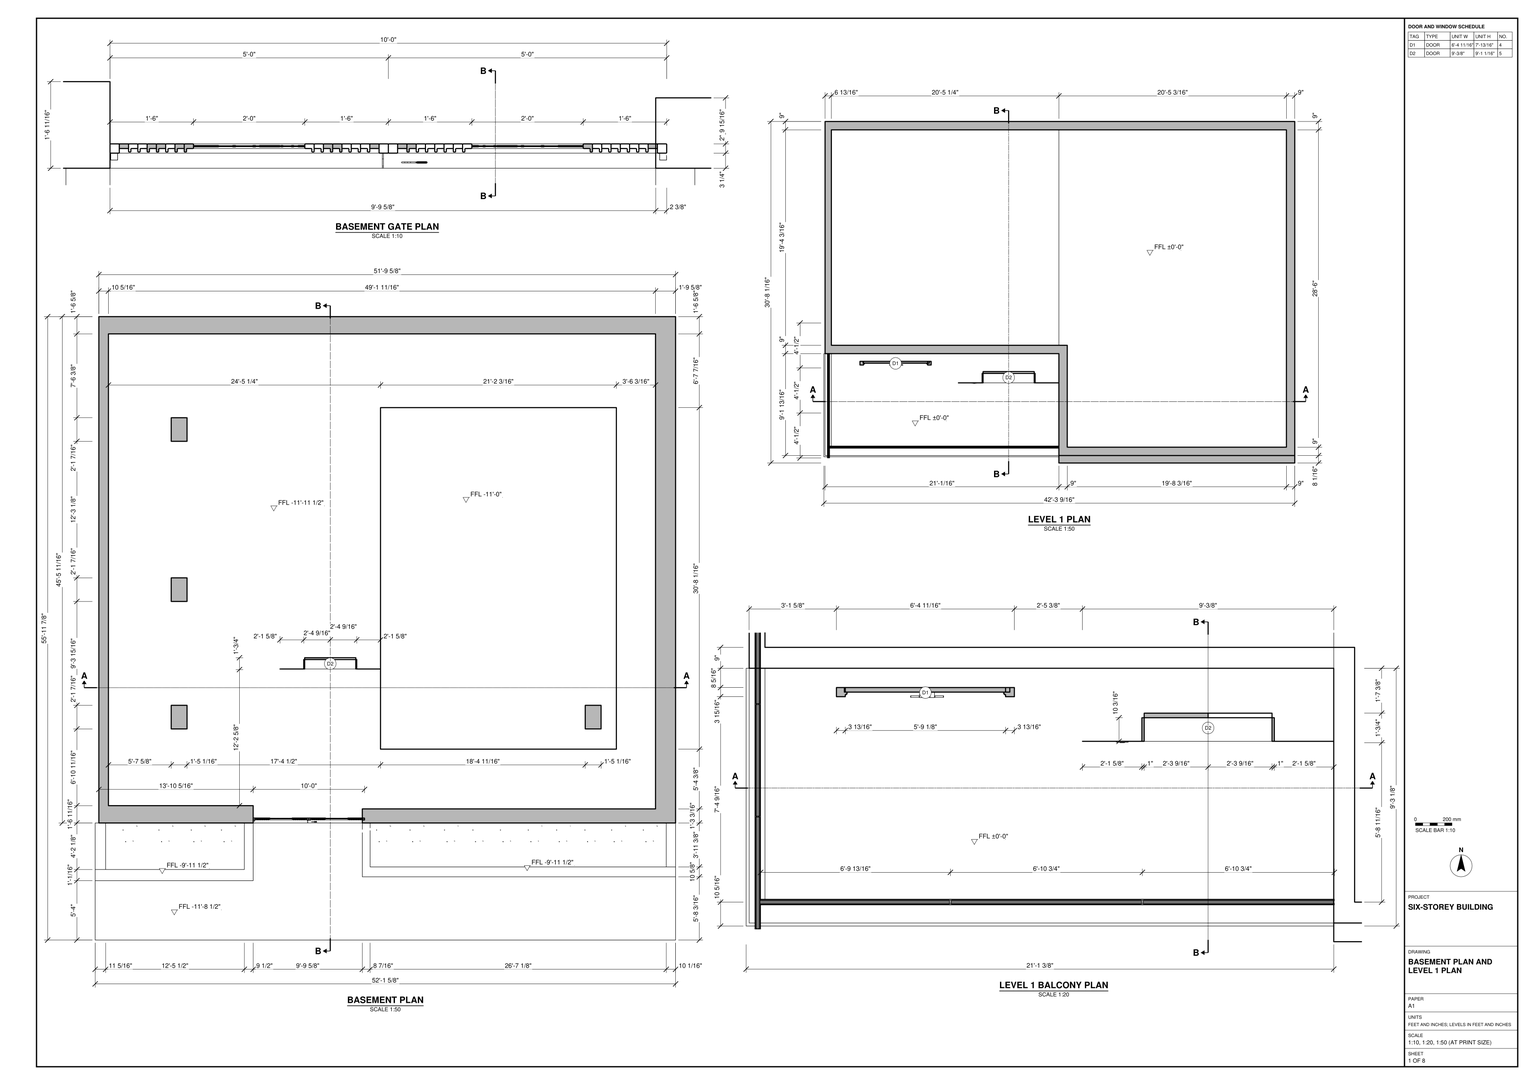
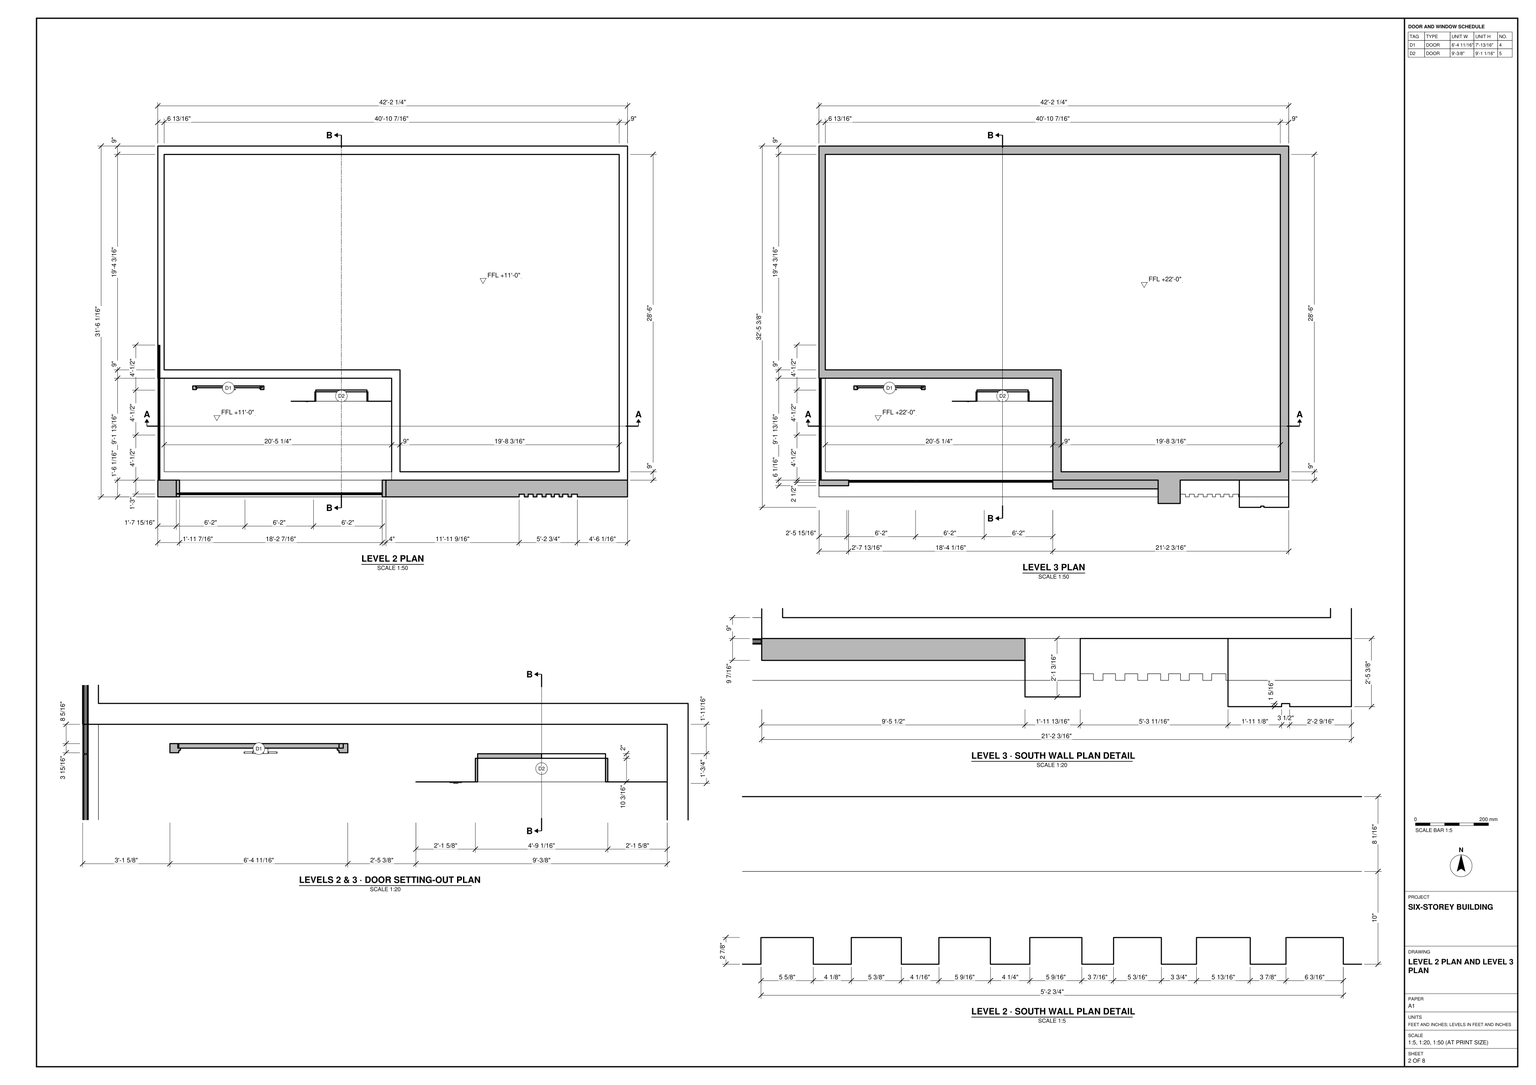
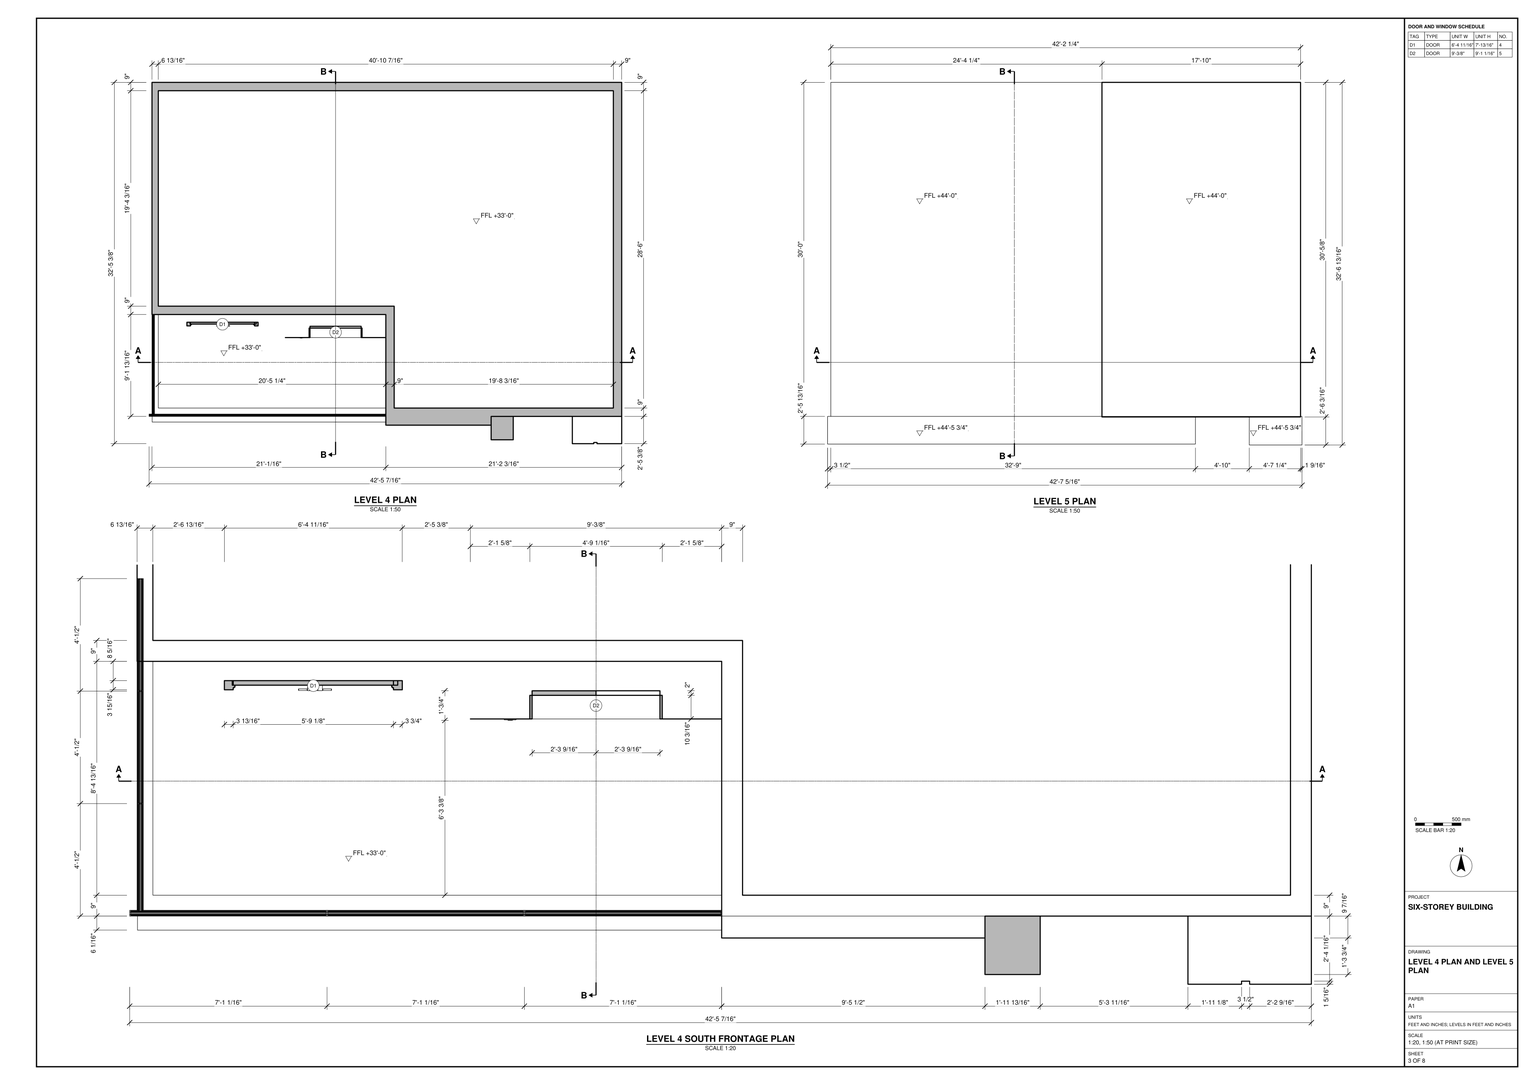
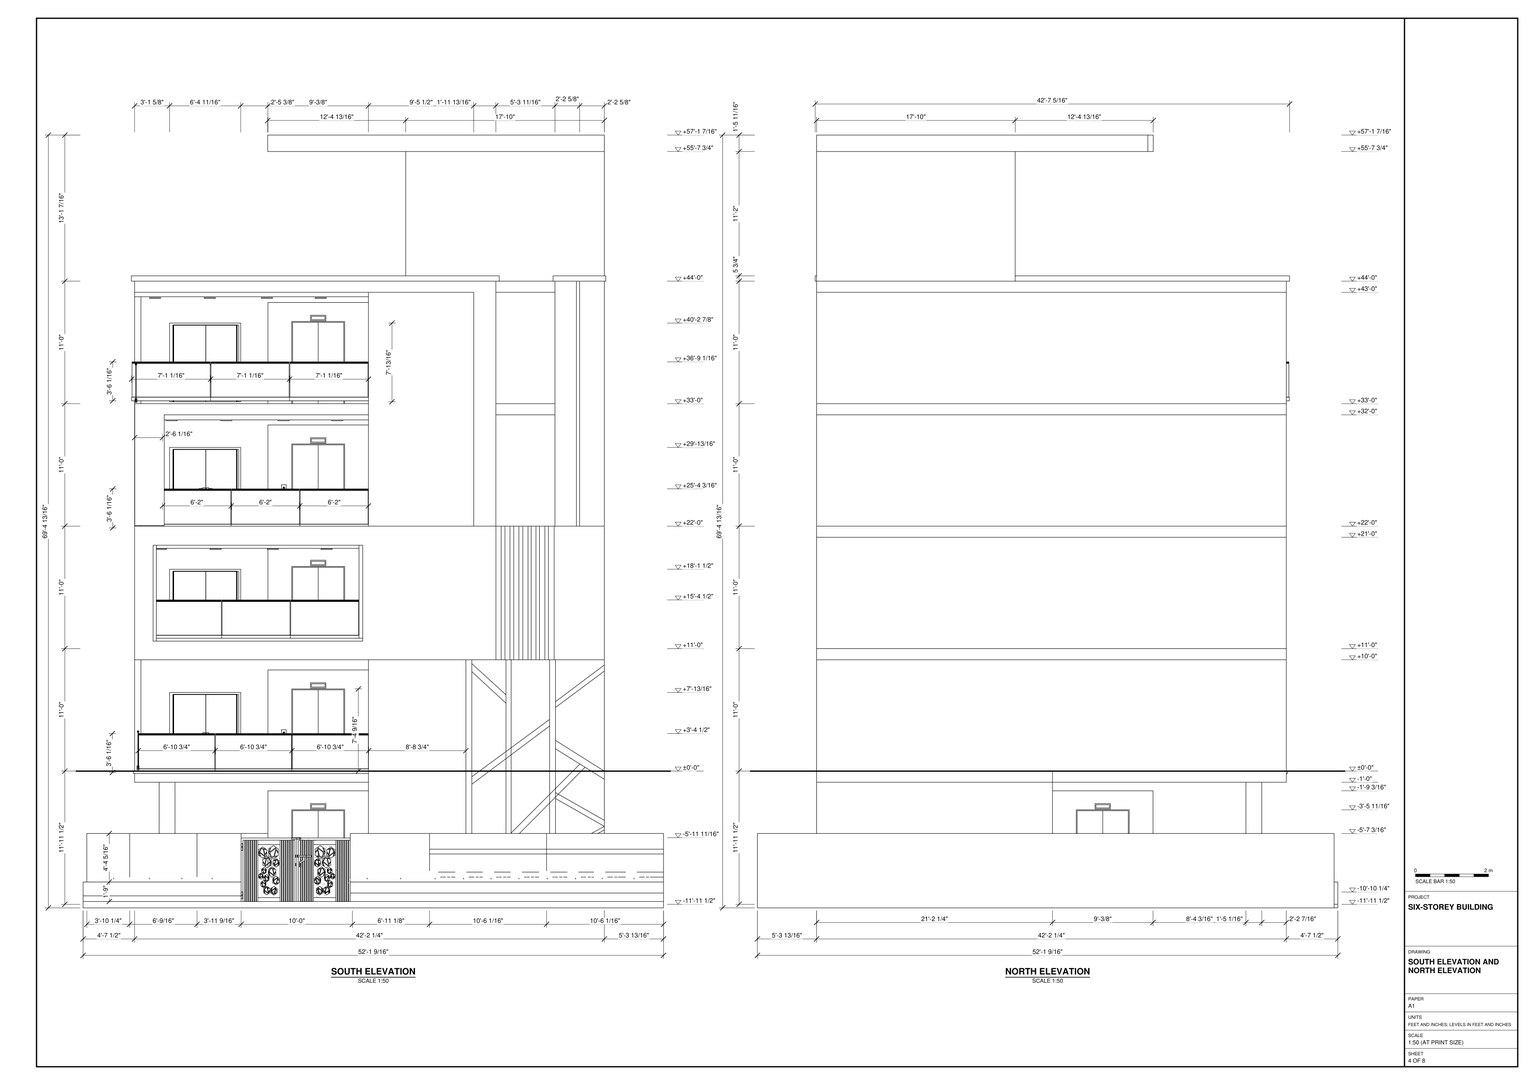
Work in feet and inches in SketchUp. Use the plans, sections, elevations and details in task_files/diagram_01.pdf. Set out the complete model at 52'-1 9/16" wide, 55'-11 7/8" deep and 69'-4 13/16" high, including the basement frontage. Use finished floor levels of -11'-11 1/2" for the basement, ±0'-0" for Level 1, +11'-0" for Level 2, +22'-0" for Level 3, +33'-0" for Level 4 and +44'-0" for Level 5.

Start with the basement perimeter, floor slabs, columns and gated opening in the south wall. Above the basement, follow the wall thicknesses and slab outlines on each plan. On Levels 1 through 4, set the balcony back into the west half of the south frontage. Place the paired entrance doors and lift doors according to the balcony details, and model the glazed balcony rails. Follow the changes in the projecting wall sections and ribbed detail on the east half of the frontage rather than copying one facade up the building. Finish the roof slabs to the outlines and heights on the Level 5 plan.

Keep shell elements such as walls, slabs and roof sections in separate groups or components, and do the same for each furniture or joinery piece shown. Use components for repeated parts. Decor and loose items may be any suitable library components. Save one SketchUp model as output_files/six_storey_building_with_recessed_balconies.skp.

# SketchUp Ruby script. Lengths in inches.
U = 1.inch
M = Sketchup.active_model
def pt(a) = Geom::Point3d.new(a.map { |v| v * U })
def face(e, loops, mat)
  f = e.add_face(loops[0].map { |a| pt(a) })
  loops[1..].each { |l| e.add_face(l.map { |a| pt(a) }).erase! }
  f.material = f.back_material = mat if mat
  f
end
# faces: each face lists its corners as indices into pts; further lists are holes
def faces(e, pts, list, mat = nil) = list.each { |f| face(e, (f[0].is_a?(Array) ? f : [f]).map { |l| l.map { |i| pts[i] } }, mat) }
# xy, xz, yz: faces in a plane at the given z, y or x. An outline is a flat list of corners, or four numbers for a rectangle; further outlines are holes
def ring(l) = l.size == 4 ? [[l[0], l[1]], [l[2], l[1]], [l[2], l[3]], [l[0], l[3]]] : l.each_slice(2).to_a
def flat(e, list, mat, &to3) = list.each { |f| face(e, (f[0].is_a?(Array) ? f : [f]).map { |l| ring(l).map { |u, v| to3.(u, v) } }, mat) }
def xy(e, z, list, mat = nil) = flat(e, list, mat) { |x, y| [x, y, z] }
def xz(e, y, list, mat = nil) = flat(e, list, mat) { |x, z| [x, y, z] }
def yz(e, x, list, mat = nil) = flat(e, list, mat) { |y, z| [x, y, z] }
def lines(e, pts, list) = list.each { |a, b| e.add_line(pt(pts[a]), pt(pts[b])) }
# prism: a flat outline (further loops are holes) pulled along v
def prism(e, loops, v, mat = nil)
  f = face(e, loops, mat); d = Geom::Vector3d.new(v.map { |x| x * U })
  f.pushpull(f.normal.samedirection?(d) ? d.length : -d.length)
end
def box(e, o, s, mat = nil) = prism(e, [[o, [o[0] + s[0], o[1], o[2]], [o[0] + s[0], o[1] + s[1], o[2]], [o[0], o[1] + s[1], o[2]]]], [0, 0, s[2]], mat)
def at(x, y, z, deg = 0) = Geom::Transformation.translation(pt([x, y, z])) * Geom::Transformation.rotation(ORIGIN, Z_AXIS, deg.degrees)
def axes(o, x, y, z) = Geom::Transformation.new([*x, 0, *y, 0, *z, 0, *pt(o).to_a, 1])
def part(name) = M.definitions.add(name)
# library, detail: a bought-in or finely detailed component or shape, given as its bounding box
def library(name, o, s) = part(name).tap { |d| box(d.entities, o, s) }
def detail(e, o, s) = box(e.add_group.entities, o, s)
def put(e, d, t, mat = nil) = e.add_instance(d, t).tap { |i| i.material = mat if mat }
def group(e, t, mat = nil) = e.add_group.tap { |g| g.transformation = t; g.material = mat if mat }.entities
root = M.entities
M.materials.add("[Color L11]").color = [153, 0, 76]
M.materials.add("[Color M06]").color = [86, 86, 86]
M.materials.add("[Color M07]").color = [58, 58, 58]
M.materials.add("[Color M08]").color = [30, 30, 30]
M.materials.add("[Color M09]").color = [0, 0, 0]
M.materials.add("[Granite Dark Gray]").color = [69, 68, 68]
M.materials.add("[Stone Brushed Khaki]").color = [226, 197, 133]
M.materials.add("[Wood Cherry Original]").color = [152, 86, 42]
M.materials.add("[Wood Veneer 01]").color = [120, 70, 37]
M.materials.add("hymenocallis littoralis").color = [156, 172, 146]
c1 = library("Elegant door(double)",[38.88,29.07,0],[76.71,4.33,84.81])
c2 = library("Building - Lift Double Door & Button",[-25.63,-1.22,0],[108.35,12.78,109.04])
c3 = library("CEILING LIGHT",[79.06,-22.11,23.17],[190.51,81.31,0.94])
c4 = library("Gate_Lasercut_10ftx6ft_Kalil",[-0.15,-3.25,-0.15],[120,5.625,60.3])
c5 = part("Group\#856")
xy(c5.entities,7.38,[[0,0,5.5,15.91]],"hymenocallis littoralis")
p = [[5.5,28.78,0],[5.5,26.79,3.44],[0,26.79,3.44],[0,28.78,0],[0,23.75,6],[5.5,23.75,6],
  [0,15.91,7.38],[5.5,15.91,7.38]]
faces(c5.entities,p,[[0,1,2,3],[4,2,1,5],[6,4,5,7]],"hymenocallis littoralis")
c6 = part("Group\#854")
xy(c6.entities,7.38,[[0,0,5.5,15.91],[0,15.91,5.5,23.87]],"hymenocallis littoralis")
p = [[5.5,31.07,4.3],[5.5,27.74,6.47],[0,27.74,6.47],[0,31.07,4.3],[0,23.87,7.38],[5.5,23.87,7.38]]
faces(c6.entities,p,[[0,1,2,3],[4,2,1,5]],"hymenocallis littoralis")
c7 = part("Group\#857")
xy(c7.entities,7.38,[[0,0,5.6,15.91]],"hymenocallis littoralis")
p = [[5.6,28.78,0],[5.6,26.79,3.44],[0,26.79,3.44],[0,28.78,0],[0,23.75,6],[5.6,23.75,6],
  [0,15.91,7.38],[5.6,15.91,7.38]]
faces(c7.entities,p,[[0,1,2,3],[4,2,1,5],[6,4,5,7]],"hymenocallis littoralis")
c8 = part("Group\#855")
put(c8.entities,c6,axes([6.09,8.57,-0.52],[0.446,0.85617,0.26089],[-0.18444,-0.19731,0.96283],[0.87582,-0.47754,0.0699]))
put(c8.entities,c6,axes([6.29,7.28,-1.71],[0.37058,0.92707,-0.05667],[-0.32382,0.19004,0.99128],[0.87712,-0.32925,0.34964]))
put(c8.entities,c6,axes([11.04,16.14,-0.7],[1,0,0],[0,0.16628,1.02662],[0,-1.18456,0.19186]))
c9 = part("Group\#860")
put(c9.entities,c5,axes([24.57,32.05,-1.76],[0.9552,-0.22102,-0.19681],[0.4036,0.95545,0.88585],[-0.00568,-0.67859,0.7345]))
put(c9.entities,c5,axes([23.95,29.24,-2.4],[0,1,0],[-0.76041,0,0.64945],[0.64945,0,0.76041]))
put(c9.entities,c5,axes([24.22,24.72,-0.48],[-0.70711,0.70711,0],[-0.32757,-0.32757,0.80237],[0.61237,0.61237,0.5]))
put(c9.entities,c6,axes([20.66,37.22,-0.63],[1.12361,0.03262,0.39091],[-0.43499,0.29739,0.78777],[0.09852,-1.27434,0.37535]))
put(c9.entities,c5,axes([28.75,24.45,-2.4],[-1,0,0],[0,-0.76041,0.64945],[0,0.64945,0.76041]))
put(c9.entities,c7,axes([30.4,30.98,-3.7],[0.65676,-0.72002,0.22414],[0.55667,0.66341,0.5],[-0.50871,-0.20361,0.83652]))
put(c9.entities,c7,axes([32.41,29.61,-3.7],[0.04029,-0.97372,0.22414],[0.85287,0.15038,0.5],[-0.52057,0.17102,0.83652]))
put(c9.entities,c5,axes([31.89,25.85,-1.76],[-0.92056,0.33739,-0.19681],[-0.5186,-0.89824,0.88585],[0.08952,0.67268,0.7345]))
put(c9.entities,c5,axes([25.55,34.78,-0.48],[0.86603,0.5,0],[-0.25,0.43301,0.86603],[0.43301,-0.75,0.5]))
put(c9.entities,c7,axes([20.4,16.9375,-8.07],[-0.70711,0.70711,0],[-0.35754,-0.35754,0.65422],[1.3987,1.3987,1.52882]))
put(c9.entities,c5,axes([32.86,34.14,-0.48],[0.76604,-0.64279,0],[0.32139,0.38302,0.86603],[-0.55667,-0.66341,0.5]))
put(c9.entities,c5,axes([27.15,34.7,-0.1],[0.82472,-0.17528,-0.53769],[0.53769,0.53769,0.64945],[0.17528,-0.82472,0.53769]))
put(c9.entities,c5,axes([33.58,28.77,-2.4],[0,-1,0],[0.76041,0,0.64945],[-0.64945,0,0.76041]))
put(c9.entities,c5,axes([26.43,23.87,-2.81],[-0.75126,0.04415,0.65853],[0.53769,-0.53769,0.64945],[0.38276,0.84199,0.3802]))
put(c9.entities,c5,axes([28.78,23.98,-2.4],[-1,0,0],[0,-0.76041,0.64945],[0,0.64945,0.76041]))
put(c9.entities,c5,axes([25.39,25.38,-2.4],[-0.70711,0.70711,0],[-0.53769,-0.53769,0.64945],[0.45923,0.45923,0.76041]))
put(c9.entities,c5,axes([27.32,21.63,-0.1],[-0.45923,0.70711,-0.53769],[-0.76041,0,0.64945],[0.45923,0.70711,0.53769]))
put(c9.entities,c5,axes([25.17,27.625,-1.76],[0.56416,0.80187,-0.19681],[-0.66673,0.66673,0.80532],[0.62659,-0.26057,0.7345]))
put(c9.entities,c7,axes([27.59,27.04,-3.96],[-0.8993,-0.06127,0.43301],[0.2962,-0.8138,0.5],[0.32175,0.57791,0.75]))
put(c9.entities,c7,axes([26.98,24.5,-3.18],[-0.5,0.86603,0],[-0.75,-0.43301,0.5],[0.43301,0.25,0.86603]))
put(c9.entities,c7,axes([24.55,27.74,-3.7],[0.29517,0.92878,0.22414],[-0.85287,0.15038,0.5],[0.43068,-0.33875,0.83652]))
put(c9.entities,c7,axes([24.26,29.8,-3.18],[0.76604,0.64279,0],[-0.47317,0.5639,0.425],[0.32139,-0.38302,0.86603]))
put(c9.entities,c7,axes([25.98,32.46,-3.18],[1,0,0],[0,0.86603,0.5],[0,-0.5,0.86603]))
put(c9.entities,c5,axes([28.78,33.57,-2.4],[1,0,0],[0,0.76041,0.64945],[0,-0.64945,0.76041]))
put(c9.entities,c8,at(14.99,21.38,2.5))
put(c9.entities,c6,axes([34.63,26.34,-1.46],[-0.70089,-0.70877,0.07994],[0.4756,-0.38088,0.79293],[-0.53156,0.59378,0.60405]))
put(c9.entities,c6,axes([28.14,16.92,1.8125],[-1.19719,0.6912,0],[-0.09607,-0.16641,0.94244],[0.68444,1.18549,0.17613]))
put(c9.entities,c6,axes([31.5625,35.84,0.97],[0.66765,-1.1564,0.35779],[0.04445,0.30732,0.91033],[-1.20828,-0.64496,0.17012]))
put(c9.entities,c6,axes([38.94,22.51,0.89],[-0.97932,-0.67164,-0.05202],[0.27787,-0.41401,0.90999],[-0.85985,0.93577,0.32097]))
put(c9.entities,c6,axes([38.44,21.09,1.98],[-1.02864,-0.54856,0.2395],[0.33481,0.06999,0.88388],[-0.77261,1.08328,0.06417]))
put(c9.entities,c7,axes([35.02,30.51,-1.3],[-0.17365,-0.98481,0],[0.60224,-0.10619,0.79122],[-0.7792,0.13739,0.61153]))
put(c9.entities,c7,axes([29.41,22.33,-1.3],[-0.93969,0.34202,0],[-0.20915,-0.57465,0.79122],[0.27061,0.74351,0.61153]))
put(c9.entities,c6,axes([19.64,36,-1.62],[1.18194,0.09546,0.08234],[-0.14377,0.68823,0.76313],[0.21457,-1.1326,0.62386]))
put(c9.entities,c7,axes([24.25,24.14,-1.3],[-0.34202,0.93969,0],[-0.57465,-0.20915,0.79122],[0.74351,0.27061,0.61153]))
put(c9.entities,c7,axes([25.98,34.61,-1.3],[1,0,0],[0,0.61153,0.79122],[0,-0.79122,0.61153]))
put(c9.entities,c7,axes([31.16,34.41,-1.64],[0.56518,-0.80224,-0.19234],[0.73413,0.34233,0.72935],[-0.47639,-0.50772,0.71782]))
put(c9.entities,c7,axes([40.52,26.84,-5.82],[-0.42262,-0.90631,0],[0.48019,-0.22391,0.68552],[-1.43418,0.66877,1.22305]))
put(c9.entities,c5,axes([29.86,38.42,-1.01],[0.89064,-0.37013,0.26413],[-0.03924,0.63286,1.01918],[-0.45353,-0.76487,0.45748]))
put(c9.entities,c5,axes([29.34,22.4,-0.48],[-0.99619,-0.08716,0],[0.04358,-0.4981,0.86603],[-0.07548,0.86273,0.5]))
c10 = part("Group\#858")
xz(c10.entities,10.07,[[9.07,0,10.07,31.01],[0,31.01,0,45.12,20.13,45.12,20.13,31.01,10.07,31.01,10.07,32.58,9.07,32.58,9.07,31.01]],"hymenocallis littoralis")
yz(c10.entities,10.07,[[0,31.01,20.13,45.12]],"hymenocallis littoralis")
p = [[9.57,9.2,0],[10.07,10.07,0],[10.07,10.07,31.01],[10.07,10.07,32.58],[9.57,9.2,32.58]]
faces(c10.entities,p,[[0,1,2,3,4]],"hymenocallis littoralis")
c11 = part("cây lá nắng")
put(c11.entities,c9,axes([49.26,-2.75,0],[0.63109,0.63109,0],[-0.63109,0.63109,0],[0,0,0.935]))
g1 = group(c11.entities,at(26.6,-8.68,0))
put(g1,c5,axes([-4.72,35.73,-1.65],[0.74231,0.46334,-0.18402],[-0.34827,0.85768,0.82827],[0.42467,-0.43184,0.68675]))
put(g1,c5,axes([-3.34,33.57,-2.24],[-0.63109,0.63109,0],[-0.47989,-0.47989,0.60723],[0.40986,0.40986,0.71098]))
put(g1,c5,axes([-0.3125,30.89,-0.45],[-0.8925,0,0],[0,-0.41345,0.75022],[0,0.77293,0.4675]))
put(g1,c6,axes([-10.79,39.66,-0.59],[0.68852,0.72969,0.3655],[-0.4622,-0.08684,0.73657],[0.86641,-0.74205,0.35095]))
put(g1,c5,axes([2.71,33.57,-2.24],[-0.63109,-0.63109,0],[0.47989,-0.47989,0.60723],[-0.40986,0.40986,0.71098]))
put(g1,c7,axes([-0.37,38.74,-3.46],[0.86887,-0.03992,0.20957],[-0.06737,0.76999,0.4675],[-0.19255,-0.44954,0.78214]))
put(g1,c7,axes([1.76,39.14,-3.46],[0.63993,-0.58908,0.20957],[0.44333,0.63315,0.4675],[-0.43646,-0.2206,0.78214]))
put(g1,c5,axes([3.81,36.4375,-1.65],[-0.79389,-0.36803,-0.18402],[0.23959,-0.89415,0.82827],[-0.36803,0.48102,0.68675]))
put(g1,c5,axes([-5.83,38.07,-0.45],[0.231,0.86209,0],[-0.43104,0.1155,0.80973],[0.74659,-0.20005,0.4675]))
put(g1,c7,axes([2.18,23.5625,-7.55],[-0.8925,0,0],[0,-0.45128,0.6117],[0,1.76542,1.42944]))
put(g1,c5,axes([-0.8125,42.28,-0.45],[0.8891,0.07779,0],[-0.03889,0.44455,0.80973],[0.06737,-0.76999,0.4675]))
put(g1,c5,axes([-4.76,39.03,-0.09],[0.63109,0.40986,-0.50274],[0,0.67866,0.60723],[0.63109,-0.40986,0.50274]))
put(g1,c5,axes([3.03,39.35,-2.24],[0.63109,-0.63109,0],[0.47989,0.47989,0.60723],[-0.40986,-0.40986,0.71098]))
put(g1,c5,axes([1.61,31.74,-2.625],[-0.50198,-0.44625,0.61573],[0.67866,0,0.60723],[-0.28982,0.77293,0.35549]))
put(g1,c5,axes([3.03,33.3,-2.24],[-0.63109,-0.63109,0],[0.47989,-0.47989,0.60723],[-0.40986,0.40986,0.71098]))
put(g1,c5,axes([0.01,32.04,-2.24],[-0.8925,0,0],[0,-0.67866,0.60723],[0,0.57963,0.71098]))
put(g1,c5,axes([3.59,30.89,-0.09],[-0.73607,0.15643,-0.50274],[-0.47989,-0.47989,0.60723],[-0.15643,0.73607,0.50274]))
put(g1,c5,axes([-1.55,33.32,-1.65],[-0.15002,0.86209,-0.18402],[-0.84154,0,0.75297],[0.55988,0.231,0.68675]))
put(g1,c7,axes([0.35,34.48,-3.71],[-0.52887,-0.60621,0.40487],[0.70051,-0.32665,0.4675],[-0.16166,0.56777,0.70125]))
put(g1,c7,axes([2.61,39.13,-1.74],[-0.86209,0.231,0],[-0.23031,-0.85954,0.15531],[0.03162,0.11799,0.91645]))
put(g1,c7,axes([-2.02,33,-3.46],[-0.39986,0.77243,0.20957],[-0.63315,-0.44333,0.4675],[0.48558,0.05802,0.78214]))
put(g1,c7,axes([-3.49,34.12,-2.97],[0.07779,0.8891,0],[-0.65449,0.05726,0.39737],[0.44455,-0.03889,0.80973]))
put(g1,c7,axes([-4.09,36.88,-2.97],[0.63109,0.63109,0],[-0.54654,0.54654,0.4675],[0.31555,-0.31555,0.80973]))
put(g1,c5,axes([-3.02,39.35,-2.24],[0.63109,0.63109,0],[-0.47989,0.47989,0.60723],[0.40986,-0.40986,0.71098]))
put(g1,c8,axes([-4.03,22.95,2.33],[0.63109,0.63109,0],[-0.63109,0.63109,0],[0,0,0.935]))
put(g1,c6,axes([5.24,38.48,-1.37],[0.00497,-0.88963,0.07474],[0.54052,0.05978,0.74139],[-0.71019,0.03927,0.56479]))
put(g1,c6,axes([7.08,28.4375,1.7],[-1.19175,-0.31933,0],[0.04439,-0.16565,0.88118],[-0.31621,1.1801,0.16468]))
put(g1,c6,axes([-2.7,42.54,0.91],[1.15114,-0.30845,0.33454],[-0.1659,0.22199,0.85115],[-0.3555,-1.16957,0.15907]))
put(g1,c6,axes([10.37,38.78,0.83],[-0.19417,-1.04191,-0.04864],[0.43664,-0.08592,0.85084],[-1.1332,0.04791,0.30011]))
put(g1,c6,axes([10.95,37.5625,1.85],[-0.30298,-0.99536,0.22393],[0.16713,0.25547,0.82643],[-1.17124,0.19607,0.06]))
put(g1,c7,axes([2.84,41.36,-1.22],[0.51192,-0.73109,0],[0.44708,0.31305,0.73979],[-0.57846,-0.40504,0.57178]))
put(g1,c7,axes([4.47,32.65,-1.22],[-0.80888,-0.37719,0],[0.23066,-0.49465,0.73979],[-0.29844,0.64,0.57178]))
put(g1,c6,axes([-10.32,35.12,-1.51],[0.68567,0.80616,0.07699],[-0.52507,0.3436,0.71352],[0.85019,-0.57936,0.58331]))
put(g1,c7,axes([0.07,30.54,-1.22],[-0.80888,0.37719,0],[-0.23066,-0.49465,0.73979],[0.29844,0.64,0.57178]))
put(g1,c7,axes([-5.45,38.24,-1.22],[0.63109,0.63109,0],[-0.38593,0.38593,0.73979],[0.49934,-0.49934,0.57178]))
put(g1,c7,axes([-2.05,41.38,-1.53],[0.86296,-0.14961,-0.17984],[0.24726,0.67935,0.68194],[0.01977,-0.62107,0.67116]))
put(g1,c7,axes([8.63,42.51,-5.4375],[0.30525,-0.83868,0],[0.44435,0.16173,0.64096],[-1.32716,-0.48305,1.14356]))
put(g1,c5,axes([-5.4,43.09,-0.94],[0.79566,0.32849,0.24696],[-0.42416,0.37462,0.95293],[0.19648,-0.76892,0.42774]))
put(g1,c5,axes([4.38,32.65,-0.45],[-0.57369,-0.68369,0],[0.34185,-0.28684,0.80973],[-0.5921,0.49683,0.4675]))
put(g1,c7,axes([-2,33.84,-0.15],[-0.24601,0.85793,0],[-0.85539,-0.24528,0.15531],[0.11742,0.03367,0.91645]))
put(g1,c7,axes([0.17,30.83,-4.47],[-0.24601,0.85793,0],[-0.85539,-0.24528,0.15531],[0.11742,0.03367,0.91645]))
put(g1,c7,axes([-1.97,32.18,-4.47],[0.58524,0.67383,0],[-0.67184,0.58351,0.15531],[0.09222,-0.0801,0.91645]))
put(g1,c7,axes([-2,34.71,-4.47],[0.88392,-0.12346,0],[0.12309,0.88131,0.15531],[-0.0169,-0.12098,0.91645]))
put(g1,c7,axes([0.11,36.12,-4.47],[0.37822,-0.8084,0],[0.80601,0.37711,0.15531],[-0.11064,-0.05177,0.91645]))
put(c11.entities,c10,axes([29.71,14.29,6.94],[0.425,0.73612,0],[-0.6771,0.39092,-0.33349],[-0.26859,0.15507,0.72712]))
put(c11.entities,c10,axes([42.0625,26.12,6.94],[0.85,0,0],[0,0.78185,-0.33349],[0,0.33349,0.78185]))
put(c11.entities,c9,axes([7.3125,23.0625,0],[0.8925,0,0],[0,0.8925,0],[0,0,0.935]))
put(c11.entities,c10,axes([24.4375,40.23,2.05],[0.85,0,0],[0,0.85,0],[0,0,0.85]))
c12 = part("Planting 101")
put(c12.entities,c11,axes([21.34,32.96,-4.59],[0,-0.71,0],[-0.71,0,0],[0,0,0.71]))
c13 = library("Wagner Glass Railing",[9.08,102.375,1.53],[2.51,145.5,42.05])
c14 = part("Group\#7")
box(c14.entities,[0,-360,0],[506.25,360,12])
c15 = part("Group\#3")
box(c15.entities,[0,0,-120],[17.0625,25.4375,120])
xy(root,-147.375,[[0,0,0,126.1875,4,126.1875,4,671.875,625.59,671.875,625.59,0]])
xy(root,-143.5,[[[170.3125,126.1875,287.95,126.1875,287.95,141.36,603.98,141.36,603.98,653.28,14.32,653.28,14.32,144.85,170.3125,144.85],[307.5625,205.75,561.78,573.8125]]])
xy(root,-140.51,[[0,0,625.59,0,625.59,68.17,287.95,68.17,287.95,126.1875,170.3125,126.1875,170.3125,64,0,64],[11.29,76.04,160.8125,126.1875],[296.38,78.8125,615.53,78.8125,615.53,126.1875,499.51,126.1875,499.51,128.8125,373.43,128.8125,373.43,126.1875,296.38,126.1875],[499.51,126.1875,625.59,128.8125]])
xy(root,-135.4,[[373.43,126.1875,499.51,128.8125],[499.51,126.1875,625.59,128.8125]])
xy(root,-134.44,[[0,64,0,76.04,160.8125,76.04,160.8125,126.1875,170.3125,126.1875,170.3125,64]])
xy(root,-132,[[307.5625,205.75,561.78,573.8125]])
xy(root,-131.38,[[287.95,68.17,287.95,126.1875,296.38,126.1875,296.38,78.8125,625.59,78.8125,625.59,68.17]])
xy(root,-119.51,[[0,64,170.3125,64,170.3125,126.1875,160.8125,126.1875,160.8125,76.04,0,76.04],[287.95,68.17,625.59,68.17,625.59,78.8125,296.38,78.8125,296.38,126.1875,287.95,126.1875],[0,76.04,11.29,126.1875],[615.53,78.8125,625.59,126.1875]])
xy(root,-114.23,[[373.43,126.1875,499.51,128.8125],[499.51,126.1875,625.59,128.8125]])
xy(root,-108.85,[[373.43,126.1875,499.51,128.8125],[499.51,126.1875,625.59,128.8125]])
xy(root,-89.28,[[373.43,126.1875,499.51,128.8125],[499.51,126.1875,625.59,128.8125]])
xy(root,-84.16,[[373.43,126.1875,499.51,128.8125],[499.51,126.1875,625.59,128.8125]])
xy(root,-67.1875,[[4,126.1875,170.3125,126.1875,170.3125,144.85,14.32,144.85,14.32,653.28,603.98,653.28,603.98,141.36,287.95,141.36,287.95,126.1875,625.59,126.1875,625.59,671.875,4,671.875]])
xy(root,-2.57,[[54.22,212.5,307.5625,213.8125],[54.22,213.8125,55.53,323.625]],"[Color M09]")
xy(root,0,[[307.5625,213.8125,561.78,213.8125,561.78,573.8125,307.5625,573.8125,307.5625,564.8125,552.78,564.8125,552.78,222.8125,316.5625,222.8125,316.5625,332.625,307.5625,332.625],[62.34,222.8125,307.5625,323.625],[316.5625,222.8125,552.78,222.8125,552.78,564.8125,307.5625,564.8125,307.5625,332.625,316.5625,332.625],[55.53,323.625,55.53,573.8125,307.5625,573.8125,307.5625,564.8125,62.34,564.8125,62.34,332.625,307.5625,332.625,307.5625,323.625],[62.34,332.625,307.5625,564.8125]])
xy(root,0,[[54.22,212.5,307.5625,212.5,307.5625,222.8125,62.34,222.8125,62.34,323.625,54.22,323.625]],"[Color M09]")
xy(root,120,[[55.53,195.75,55.53,213.8125,307.5625,213.8125,307.5625,205.75,561.78,205.75,561.78,195.75,507.72,195.75,507.72,198.625,501.54,198.625,501.54,195.75,497.69,195.75,497.69,198.625,491.9,198.625,491.9,195.75,488.11,195.75,488.11,198.625,482.96,198.625,482.96,195.75,479.54,195.75,479.54,198.625,473.93,198.625,473.93,195.75,469.68,195.75,469.68,198.625,464.13,198.625,464.13,195.75,460.09,195.75,460.09,198.625,454.69,198.625,454.69,195.75,450.6,195.75,450.6,198.625,444.95,198.625,444.95,195.75],[307.5625,205.75,561.78,213.8125],[[307.5625,213.8125,561.78,213.8125,561.78,573.8125,55.53,573.8125,55.53,323.625,307.5625,323.625],[316.5625,222.8125,316.5625,332.625,62.34,332.625,62.34,564.8125,552.78,564.8125,552.78,222.8125]]])
xy(root,132,[[55.53,213.8125,307.5625,213.8125,307.5625,222.8125,62.34,222.8125,62.34,323.625,55.53,323.625],[[307.5625,213.8125,307.5625,323.625,55.53,323.625,55.53,573.8125,561.78,573.8125,561.78,213.8125],[316.5625,222.8125,552.78,222.8125,552.78,564.8125,62.34,564.8125,62.34,332.625,316.5625,332.625]],[316.5625,222.8125,552.78,222.8125,552.78,564.8125,62.34,564.8125,62.34,332.625,316.5625,332.625],[62.34,222.8125,307.5625,323.625]])
xy(root,140.0625,[[75.44,195.75,78.94,213.8125],[78.94,195.75,301.38,213.8125]])
xy(root,143.1875,[[78.94,195.75,297.38,213.8125],[297.38,195.75,301.38,213.8125]])
xy(root,240.0625,[[78.94,195.75,297.38,213.8125]])
xy(root,243.4375,[[75.44,195.75,78.94,213.8125],[78.94,195.75,297.38,213.8125],[297.38,195.75,301.38,213.8125]])
xy(root,246,[[55.53,230.07,307.5625,321.17]],"[Wood Cherry Original]")
xy(root,252,[[[307.5625,213.8125,561.78,213.8125,561.78,573.8125,55.53,573.8125,55.53,323.625,307.5625,323.625],[316.5625,222.8125,316.5625,332.625,62.34,332.625,62.34,564.8125,552.78,564.8125,552.78,222.8125]],[55.53,230.07,307.5625,321.17]])
xy(root,264,[[508.59,184.4375,508.59,195.75,561.78,195.75,561.78,184.4375,535.18,184.4375,535.18,185.75,531.6875,185.75,531.6875,184.4375],[421.07,188.625,444.88,195.75],[55.53,195.75,421.07,195.75,421.07,204.375,307.5625,204.375,307.5625,213.8125,55.53,213.8125],[421.07,195.75,444.88,213.8125],[444.88,195.75,444.95,195.75,444.95,198.625,450.6,198.625,450.6,195.75,454.69,195.75,454.69,198.625,460.09,198.625,460.09,195.75,464.13,195.75,464.13,198.625,469.68,198.625,469.68,195.75,473.93,195.75,473.93,198.625,479.54,198.625,479.54,195.75,482.96,195.75,482.96,198.625,488.11,198.625,488.11,195.75,491.9,195.75,491.9,198.625,497.69,198.625,497.69,195.75,501.54,195.75,501.54,198.625,507.72,198.625,507.72,195.75,508.59,195.75,508.59,213.8125,444.88,213.8125],
  [508.59,195.75,561.78,213.8125],[55.53,213.8125,307.5625,213.8125,307.5625,222.8125,62.34,222.8125,62.34,323.625,55.53,323.625],[[307.5625,213.8125,307.5625,323.625,55.53,323.625,55.53,573.8125,561.78,573.8125,561.78,213.8125],[316.5625,222.8125,552.78,222.8125,552.78,564.8125,62.34,564.8125,62.34,332.625,316.5625,332.625]],[316.5625,222.8125,552.78,222.8125,552.78,564.8125,62.34,564.8125,62.34,332.625,316.5625,332.625],[62.34,222.8125,307.5625,323.625]])
xy(root,264.625,[[55.7,207.75,87.49,213.8125]])
xy(root,378.5,[[55.53,222.8125,307.5625,323.625]],"[Wood Cherry Original]")
xy(root,384,[[[307.5625,213.8125,561.78,213.8125,561.78,573.8125,55.53,573.8125,55.53,323.625,307.5625,323.625],[316.5625,222.8125,316.5625,332.625,62.34,332.625,62.34,564.8125,552.78,564.8125,552.78,222.8125]]])
xy(root,384,[[87.49,207.75,307.5625,213.8125]],"[Color M06]")
xy(root,396,[[[307.5625,213.8125,307.5625,323.625,55.53,323.625,55.53,573.8125,561.78,573.8125,561.78,213.8125],[316.5625,222.8125,552.78,222.8125,552.78,564.8125,62.34,564.8125,62.34,332.625,316.5625,332.625]],[316.5625,222.8125,552.78,222.8125,552.78,564.8125,62.34,564.8125,62.34,332.625,316.5625,332.625],[62.34,222.8125,307.5625,323.625]])
xy(root,396,[[55.7,207.75,55.7,213.8125,55.53,213.8125,55.53,323.625,62.34,323.625,62.34,222.8125,307.5625,222.8125,307.5625,207.75]],"[Color M06]")
xy(root,511.25,[[55.53,204.375,307.5625,323.625]],"[Wood Cherry Original]")
xy(root,516,[[55.53,188.625,421.07,204.375],[307.5625,204.375,421.07,213.8125],[[307.5625,213.8125,561.78,213.8125,561.78,573.8125,55.53,573.8125,55.53,323.625,307.5625,323.625],[316.5625,222.8125,316.5625,332.625,62.34,332.625,62.34,564.8125,552.78,564.8125,552.78,222.8125]]])
xy(root,528,[[506.52,183,506.52,184.4375,531.6875,184.4375,531.6875,185.75,535.18,185.75,535.18,184.4375,563.34,184.4375,563.34,183],[52.03,184,52.03,213.8125,55.53,213.8125,55.53,188.625,444.88,188.625,444.88,213.21,448.51,213.21,448.51,184],[506.52,184.4375,508.59,213.21],[508.59,184.4375,508.59,213.21,561.78,213.21,561.78,184.4375,535.18,184.4375,535.18,185.75,531.6875,185.75,531.6875,184.4375],[561.78,184.4375,563.34,213.8125],
  [55.53,188.625,55.53,213.8125,347.76,213.8125,347.76,213.21,444.88,213.21,444.88,188.625],[347.76,213.21,444.88,213.8125],[448.51,213.21,448.51,213.8125,347.76,213.8125,347.76,573.8125,561.78,573.8125,561.78,213.8125,506.52,213.8125,506.52,213.21],[444.88,213.21,448.51,213.8125],[506.52,213.21,508.59,213.8125],
  [508.59,213.21,561.78,213.8125]])
xy(root,533.75,[[506.52,183,563.34,213.8125],[52.03,184,448.51,213.8125]],"[Granite Dark Gray]")
xy(root,667.75,[[347.76,213.21,561.78,573.8125]])
xy(root,667.75,[[198.95,171.64,561.78,181.33],[198.95,181.33,204.76,573.8125]],"[Color M08]")
xy(root,667.75,[[204.76,181.33,204.76,573.8125,347.76,573.8125,347.76,213.21,561.78,213.21,561.78,181.33]],"[Wood Cherry Original]")
xy(root,685.4375,[[204.76,181.33,561.78,573.8125]])
xy(root,685.4375,[[198.95,171.64,561.78,181.33],[198.95,181.33,204.76,573.8125]],"[Color M08]")
xz(root,0,[[0,-147.375,625.59,-140.51]])
xz(root,64,[[0,-140.51,170.3125,-134.44]])
xz(root,64,[[0,-134.44,170.3125,-119.51]],"[Color L11]")
xz(root,68.17,[[287.95,-140.51,625.59,-131.38]])
xz(root,68.17,[[287.95,-131.38,625.59,-119.51]],"[Color L11]")
xz(root,76.04,[[11.29,-140.51,160.8125,-134.44],[0,-134.44,11.29,-119.51],[11.29,-134.44,160.8125,-119.51]])
xz(root,78.8125,[[296.38,-140.51,615.53,-131.38],[296.38,-131.38,615.53,-119.51],[615.53,-131.38,625.59,-119.51]])
xz(root,126.1875,[[0,-147.375,4,-143.5],[0,-143.5,4,-119.51],[4,-143.5,170.3125,-143.5,170.3125,-134.44,160.8125,-134.44,160.8125,-140.51,11.29,-140.51,11.29,-119.51,4,-119.51],[170.3125,-143.5,287.95,-140.51],[11.29,-140.51,50.23,-140.51,50.23,-67.1875,4,-67.1875,4,-119.51,11.29,-119.51],
  [50.23,-140.51,122.76,-67.1875],[122.76,-140.51,160.8125,-140.51,160.8125,-119.51,170.3125,-119.51,170.3125,-67.1875,122.76,-67.1875],[296.38,-140.51,373.43,-140.51,373.43,-67.1875,287.95,-67.1875,287.95,-119.51,296.38,-119.51],[615.53,-140.51,625.59,-135.4],[373.43,-135.4,499.51,-114.23],
  [160.8125,-134.44,170.3125,-119.51],[287.95,-131.38,296.38,-119.51],[373.43,-108.85,499.51,-89.28],[373.43,-84.16,499.51,-67.1875]])
xz(root,126.1875,[[499.51,-135.4,615.53,-135.4,615.53,-119.51,625.59,-119.51,625.59,-114.23,499.51,-114.23],[615.53,-135.4,625.59,-119.51],[499.51,-108.85,625.59,-89.28],[499.51,-84.16,625.59,-67.1875]],"[Color M07]")
xz(root,128.8125,[[499.51,-140.51,625.59,-135.4],[499.51,-114.23,625.59,-108.85],[499.51,-89.28,625.59,-84.16]])
xz(root,128.8125,[[373.43,-140.51,499.51,-135.4],[373.43,-114.23,499.51,-108.85],[373.43,-89.28,499.51,-84.16]],"[Color M07]")
xz(root,141.36,[[287.95,-143.5,603.98,-67.1875]])
xz(root,144.85,[[14.32,-143.5,170.3125,-67.1875]])
xz(root,171.64,[[198.95,667.75,561.78,685.4375]],"[Color M08]")
xz(root,181.33,[[198.95,667.75,204.76,685.4375],[204.76,667.75,561.78,685.4375]])
xz(root,183,[[506.52,528,563.34,533.75]],"[Granite Dark Gray]")
xz(root,184,[[52.03,528,448.51,533.75]],"[Granite Dark Gray]")
xz(root,184.4375,[[508.59,264,531.6875,528],[535.18,264,561.78,528]])
xz(root,185.75,[[531.6875,264,535.18,528]])
xz(root,188.625,[[421.07,264,444.88,264,444.88,528,55.53,528,55.53,516,421.07,516]])
xz(root,195.75,[[[55.53,120,444.95,264],[75.44,140.0625,301.38,243.4375]],[450.6,120,454.69,264],[460.09,120,464.13,264],[469.68,120,473.93,264],[479.54,120,482.96,264],
  [488.11,120,491.9,264],[497.69,120,501.54,264],[507.72,120,561.78,264]])
xz(root,195.75,[[75.44,140.0625,78.94,243.4375],[78.94,140.0625,301.38,143.1875],[297.38,143.1875,301.38,243.4375],[78.94,240.0625,297.38,243.4375]],"[Color M08]")
xz(root,198.625,[[444.95,120,450.6,264],[454.69,120,460.09,264],[464.13,120,469.68,264],[473.93,120,479.54,264],[482.96,120,488.11,264],
  [491.9,120,497.69,264],[501.54,120,507.72,264]],"[Granite Dark Gray]")
xz(root,204.375,[[307.5625,264,421.07,516]])
xz(root,204.375,[[55.53,511.25,307.5625,516]],"[Wood Cherry Original]")
xz(root,205.75,[[307.5625,-143.5,412.59,-132],[412.59,-143.5,418.96,-132],[418.96,-143.5,455.77,-132],[455.77,-143.5,461.34,-132],[461.34,-143.5,474.51,-132],
  [474.51,-143.5,502.84,-132],[502.84,-143.5,509.15,-132],[509.15,-143.5,561.78,-132],[307.5625,-132,412.59,120],[418.96,-132,455.77,-132,455.77,-107.62,418.96,-80.99],
  [461.34,-132,502.84,-97.68,502.84,-34.31,461.34,-76.2],[474.51,-132,502.84,-132,502.84,-107.62],[509.15,-132,561.78,-132,561.78,-63.35,509.15,-92.77],[455.77,-97.68,455.77,13.43,418.96,-14.11,418.96,-73.06],[509.15,-88.46,561.78,-59.52,509.15,-29.45],
  [461.34,-66.64,502.84,-25.0625,502.84,48.65,461.34,17.59],[561.78,-53,561.78,-8.79,540.97,4.19,512.2,-24.85],[509.15,-18.74,535.47,7.625,509.15,24.04],[418.96,-6,455.77,21.09,455.77,73.22,418.96,107.22],[561.78,0,561.78,107.78,509.15,68.61,509.15,33.12],
  [461.34,25.1875,502.84,55.73,502.84,120,461.34,120],[509.15,74.83,561.78,114.4,561.78,120,509.15,120],[455.77,82.24,455.77,120,418.96,120,418.96,115.86]])
xz(root,205.75,[[412.59,-132,418.96,120],[455.77,-132,461.34,-132,461.34,17.59,455.77,13.43],[461.34,-132,474.51,-132,502.84,-107.62,502.84,-97.68],[502.84,-132,509.15,-132,509.15,-27.93,502.84,-34.31],[455.77,-107.62,455.77,-97.68,418.96,-73.06,418.96,-80.99],
  [509.15,-92.77,561.78,-63.35,561.78,-59.52,509.15,-88.46],[461.34,-76.2,502.84,-34.31,502.84,-25.0625,461.34,-66.64],[561.78,-59.52,561.78,-53,512.2,-24.85,509.15,-27.93,509.15,-29.45],[502.84,-34.31,509.15,-27.93,509.15,-18.74,502.84,-25.0625],[509.15,-27.93,512.2,-24.85,509.15,-23.12],
  [502.84,-25.0625,509.15,-18.74,509.15,120,502.84,120],[512.2,-24.85,540.97,4.19,535.47,7.625,509.15,-18.74,509.15,-23.12],[418.96,-14.11,455.77,13.43,455.77,21.09,418.96,-6],[561.78,-8.79,561.78,0,509.15,33.12,509.15,24.04,535.47,7.625,540.97,4.19],[455.77,13.43,461.34,17.59,461.34,25.1875,455.77,21.09],
  [461.34,17.59,502.84,48.65,502.84,55.73,461.34,25.1875],[455.77,21.09,461.34,25.1875,461.34,120,455.77,120],[509.15,68.61,561.78,107.78,561.78,114.4,509.15,74.83],[455.77,73.22,455.77,82.24,418.96,115.86,418.96,107.22]],"[Stone Brushed Khaki]")
xz(root,207.75,[[55.7,264.625,87.49,264.625,87.49,384,307.5625,384,307.5625,396,55.7,396]],"[Color M06]")
xz(root,212.5,[[54.22,-2.57,307.5625,0]],"[Color M09]")
xz(root,213.21,[[347.76,528,561.78,667.75]])
xz(root,213.8125,[[307.5625,0,561.78,120],[55.53,120,307.5625,132],[307.5625,120,561.78,132],[[55.53,132,55.53,264,307.5625,264,307.5625,252,561.78,252,561.78,132],[75.44,140.0625,301.38,243.4375]],[75.44,140.0625,78.94,243.4375],
  [78.94,140.0625,301.38,143.1875],[297.38,143.1875,301.38,243.4375],[78.94,240.0625,297.38,243.4375],[307.5625,252,561.78,264],[307.5625,264,421.07,384],
  [508.59,264,561.78,384],[307.5625,384,421.07,396],[421.07,384,444.88,396],[508.59,384,561.78,396],[421.07,396,444.88,516],
  [508.59,396,561.78,516],[508.59,516,561.78,528]])
xz(root,213.8125,[[55.7,264.625,55.7,396,307.5625,396,307.5625,384,87.49,384,87.49,264.625]],"[Color M06]")
xz(root,213.8125,[[52.03,528,448.51,533.75],[506.52,528,563.34,533.75]],"[Granite Dark Gray]")
xz(root,213.8125,[[444.88,264,508.59,384],[444.88,384,508.59,396],[444.88,396,508.59,516]],"[Wood Veneer 01]")
xz(root,222.8125,[[316.5625,0,552.78,120],[316.5625,132,552.78,252],[316.5625,264,552.78,384],[316.5625,396,552.78,516]])
xz(root,222.8125,[[55.53,378.5,307.5625,384]],"[Wood Cherry Original]")
xz(root,230.07,[[55.53,246,307.5625,252]],"[Wood Cherry Original]")
xz(root,321.17,[[55.53,246,307.5625,252]])
xz(root,323.625,[[54.22,-2.57,55.53,0],[55.53,0,62.34,120],[62.34,0,307.5625,120],[55.53,132,62.34,252],[62.34,132,307.5625,252],
  [55.53,264,62.34,378.5],[62.34,264,307.5625,378.5],[55.53,378.5,62.34,384],[62.34,378.5,307.5625,384],[55.53,396,62.34,511.25],
  [62.34,396,307.5625,511.25],[55.53,511.25,62.34,516],[62.34,511.25,307.5625,516]])
xz(root,332.625,[[62.34,0,316.5625,120],[62.34,132,316.5625,252],[62.34,264,316.5625,384],[62.34,396,316.5625,516]])
xz(root,564.8125,[[62.34,0,552.78,120],[62.34,132,552.78,252],[62.34,264,552.78,384],[62.34,396,552.78,516]])
xz(root,573.8125,[[307.5625,-143.5,561.78,-132],[307.5625,-132,561.78,0],[55.53,0,561.78,120],[55.53,132,561.78,252],[55.53,264,561.78,384],
  [55.53,396,561.78,516],[347.76,528,561.78,667.75],[198.95,667.75,204.76,685.4375],[204.76,667.75,561.78,685.4375]])
xz(root,653.28,[[14.32,-143.5,603.98,-67.1875]])
xz(root,671.875,[[4,-147.375,625.59,-67.1875]])
yz(root,0,[[0,-147.375,0,-140.51,64,-140.51,64,-134.44,76.04,-134.44,76.04,-119.51,126.1875,-119.51,126.1875,-147.375],[64,-134.44,76.04,-119.51]])
yz(root,4,[[126.1875,-147.375,671.875,-67.1875]])
yz(root,11.29,[[76.04,-140.51,126.1875,-119.51]])
yz(root,14.32,[[144.85,-143.5,653.28,-67.1875]])
yz(root,52.03,[[184,528,213.8125,533.75]],"[Granite Dark Gray]")
yz(root,54.22,[[212.5,-2.57,213.8125,0],[213.8125,-2.57,323.625,0]],"[Color M09]")
yz(root,55.53,[[323.625,0,573.8125,120],[195.75,120,213.8125,264],[323.625,132,573.8125,252],[323.625,264,573.8125,384],[323.625,396,573.8125,516],
  [188.625,516,213.8125,528]])
yz(root,55.53,[[230.07,246,321.17,252],[222.8125,378.5,323.625,384],[204.375,511.25,323.625,516]],"[Wood Cherry Original]")
yz(root,55.7,[[207.75,264.625,213.8125,396]],"[Color M06]")
yz(root,62.34,[[332.625,0,564.8125,120],[332.625,132,564.8125,252],[332.625,264,564.8125,384],[332.625,396,564.8125,516]])
yz(root,75.44,[[195.75,140.0625,213.8125,243.4375]])
yz(root,78.94,[[195.75,140.0625,213.8125,143.1875],[195.75,143.1875,213.8125,240.0625],[195.75,240.0625,213.8125,243.4375]])
yz(root,87.49,[[207.75,264.625,213.8125,384]],"[Color M06]")
yz(root,160.8125,[[76.04,-140.51,126.1875,-134.44],[76.04,-134.44,126.1875,-119.51]])
yz(root,170.3125,[[126.1875,-143.5,144.85,-67.1875],[64,-140.51,126.1875,-134.44]])
yz(root,170.3125,[[64,-134.44,126.1875,-119.51]],"[Color L11]")
yz(root,198.95,[[171.64,667.75,181.33,685.4375],[181.33,667.75,573.8125,685.4375]],"[Color M08]")
yz(root,204.76,[[181.33,667.75,573.8125,685.4375]])
yz(root,287.95,[[126.1875,-143.5,141.36,-67.1875],[68.17,-140.51,126.1875,-131.38]])
yz(root,287.95,[[68.17,-131.38,126.1875,-119.51]],"[Color L11]")
yz(root,296.38,[[78.8125,-140.51,126.1875,-131.38],[78.8125,-131.38,126.1875,-119.51]])
yz(root,297.38,[[195.75,143.1875,213.8125,240.0625],[195.75,240.0625,213.8125,243.4375]])
yz(root,301.38,[[195.75,140.0625,213.8125,143.1875],[195.75,143.1875,213.8125,243.4375]])
yz(root,307.5625,[[205.75,-143.5,212.5,-132],[212.5,-143.5,573.8125,-132],[205.75,-132,212.5,0],[212.5,-132,573.8125,-2.57],[212.5,-2.57,573.8125,0],
  [205.75,0,213.8125,120],[213.8125,0,222.8125,120],[222.8125,0,323.625,120],[222.8125,132,222.8125,252,230.07,252,230.07,246,321.17,246,321.17,252,323.625,252,323.625,132],[230.07,246,321.17,252],
  [204.375,264,204.375,511.25,213.8125,511.25,213.8125,396,207.75,396,207.75,384,213.8125,384,213.8125,264],[213.8125,264,222.8125,384],[222.8125,264,323.625,378.5],[222.8125,378.5,323.625,384],[207.75,384,213.8125,396],
  [213.8125,396,222.8125,511.25],[222.8125,396,323.625,511.25],[204.375,511.25,323.625,516]])
yz(root,316.5625,[[222.8125,0,332.625,120],[222.8125,132,332.625,252],[222.8125,264,332.625,384],[222.8125,396,332.625,516]])
yz(root,347.76,[[213.21,528,573.8125,667.75]])
yz(root,373.43,[[126.1875,-140.51,128.8125,-135.4],[126.1875,-114.23,128.8125,-108.85],[126.1875,-89.28,128.8125,-84.16]])
yz(root,421.07,[[188.625,264,204.375,516],[204.375,264,213.8125,516]])
yz(root,444.88,[[188.625,264,213.8125,528]])
yz(root,444.95,[[195.75,120,198.625,264]])
yz(root,448.51,[[184,528,213.8125,533.75]],"[Granite Dark Gray]")
yz(root,450.6,[[195.75,120,198.625,264]])
yz(root,454.69,[[195.75,120,198.625,264]])
yz(root,460.09,[[195.75,120,198.625,264]])
yz(root,464.13,[[195.75,120,198.625,264]])
yz(root,469.68,[[195.75,120,198.625,264]])
yz(root,473.93,[[195.75,120,198.625,264]])
yz(root,479.54,[[195.75,120,198.625,264]])
yz(root,482.96,[[195.75,120,198.625,264]])
yz(root,488.11,[[195.75,120,198.625,264]])
yz(root,491.9,[[195.75,120,198.625,264]])
yz(root,497.69,[[195.75,120,198.625,264]])
yz(root,501.54,[[195.75,120,198.625,264]])
yz(root,506.52,[[183,528,213.8125,533.75]],"[Granite Dark Gray]")
yz(root,507.72,[[195.75,120,198.625,264]])
yz(root,508.59,[[184.4375,264,213.8125,528]])
yz(root,531.6875,[[184.4375,264,185.75,528]])
yz(root,535.18,[[184.4375,264,185.75,528]])
yz(root,552.78,[[222.8125,0,564.8125,120],[222.8125,132,564.8125,252],[222.8125,264,564.8125,384],[222.8125,396,564.8125,516]])
yz(root,561.78,[[205.75,-143.5,573.8125,-132],[205.75,-132,573.8125,0],[205.75,0,213.8125,120],[213.8125,0,573.8125,120],[195.75,120,213.8125,264],
  [213.8125,132,573.8125,252],[184.4375,264,213.8125,528],[213.8125,264,573.8125,384],[213.8125,396,573.8125,516],[213.21,528,573.8125,667.75],
  [171.64,667.75,181.33,685.4375],[181.33,667.75,573.8125,685.4375]])
yz(root,563.34,[[183,528,213.8125,533.75]],"[Granite Dark Gray]")
yz(root,603.98,[[141.36,-143.5,653.28,-67.1875]])
yz(root,615.53,[[78.8125,-140.51,126.1875,-119.51]])
yz(root,625.59,[[0,-147.375,126.1875,-147.375,126.1875,-119.51,78.8125,-119.51,78.8125,-131.38,68.17,-131.38,68.17,-140.51,0,-140.51],[126.1875,-147.375,671.875,-147.375,671.875,-67.1875,126.1875,-67.1875,126.1875,-84.16,128.8125,-84.16,128.8125,-89.28,126.1875,-89.28,126.1875,-108.85,128.8125,-108.85,128.8125,-114.23,126.1875,-114.23,126.1875,-135.4,128.8125,-135.4,128.8125,-140.51,126.1875,-140.51],[68.17,-131.38,78.8125,-119.51]])
put(root,c1,at(54.28,281.91,0))
put(root,c1,at(54.28,281.91,132.6875))
put(root,c1,at(54.28,281.91,264))
put(root,c2,at(224.85,292.72,0))
put(root,c2,at(224.85,299.39,132))
put(root,c2,at(224.85,299.39,264))
put(root,c2,at(224.85,299.39,396))
put(root,c1,at(54.28,281.91,398.0625))
put(root,c3,at(-7.46,250.23,486.21))
put(root,c3,at(10.41,256.6,354.39))
put(root,c3,at(-1.16,259.01,215.64))
put(root,c2,at(224.85,292.72,-130.25))
put(root,c4,axes([170.46,129.4375,-143.28],[1,0,0],[0,1,0],[0,0,1.19]))
put(root,c12,at(316.49,108.77,-131.51))
put(root,c12,at(352.55,108.77,-131.51))
put(root,c12,at(389.68,108.77,-131.51))
put(root,c12,at(420.3,108.77,-131.51))
put(root,c12,at(449.99,108.77,-131.51))
put(root,c12,at(479.99,108.77,-131.51))
put(root,c12,at(510.55,108.77,-131.51))
put(root,c12,at(541.05,108.77,-131.51))
put(root,c12,at(569.8,108.77,-131.51))
put(root,c12,at(603.99,108.77,-131.51))
put(root,c12,at(149.3,108.77,-131.51))
put(root,c12,at(116.74,108.77,-131.51))
put(root,c12,at(81.93,108.77,-131.51))
put(root,c12,at(43.24,108.77,-131.51))
put(root,c13,at(48.89,108.81,0))
put(root,c13,axes([-115.2,233.18,-3.06],[0,-1,0],[1.70657,0,0],[0,0,1]))
put(root,c13,axes([-80.72,209.42,140.89],[0,-1,0],[1.52534,0,0],[0,0,1]))
put(root,c13,axes([-70.53,222.89,260.59],[0,-1,0],[1.52534,0,0],[0,0,1]))
put(root,c13,axes([-127.25,225.41,397.51],[0,-1,0],[1.75415,0,0],[0,0,1]))
put(root,c13,at(46.45,111.4375,130.49))
put(root,c13,at(46.625,111.4375,266.98))
put(root,c13,at(46.625,111.4375,395.81))
put(root,c14,at(55.53,573.8125,-12))
put(root,c14,at(55.53,573.8125,120))
put(root,c14,at(55.53,573.8125,252))
g2 = group(root,at(55.53,573.8125,384))
box(g2,[0,-360,0],[506.25,360,12])
put(root,c15,at(528.22,227.54,-12))
g3 = group(root,at(55.53,573.8125,516))
box(g3,[0,-360,0],[506.25,360,12])
put(root,c15,at(81.97,227.54,-12))
put(root,c15,at(81.97,364.92,-12))
put(root,c15,at(81.97,537.48,-12))
